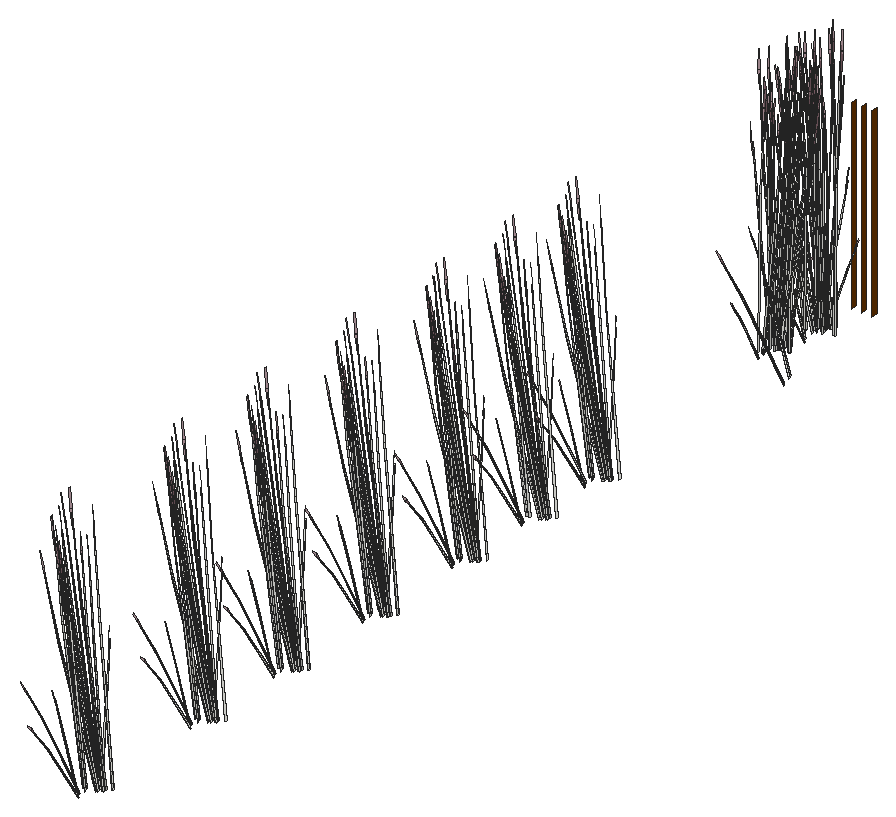
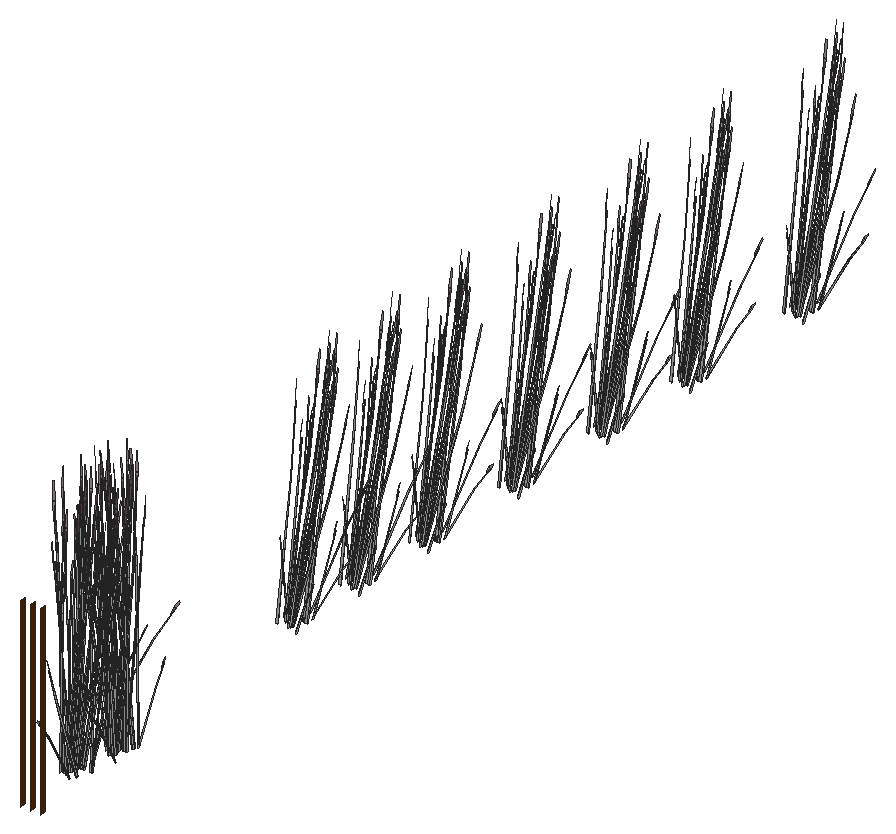
# SketchUp Ruby script. Lengths in inches.
U = 1.inch
M = Sketchup.active_model
def pt(a) = Geom::Point3d.new(a.map { |v| v * U })
def face(e, loops, mat)
  f = e.add_face(loops[0].map { |a| pt(a) })
  loops[1..].each { |l| e.add_face(l.map { |a| pt(a) }).erase! }
  f.material = f.back_material = mat if mat
  f
end
# faces: each face lists its corners as indices into pts; further lists are holes
def faces(e, pts, list, mat = nil) = list.each { |f| face(e, (f[0].is_a?(Array) ? f : [f]).map { |l| l.map { |i| pts[i] } }, mat) }
# xy, xz, yz: faces in a plane at the given z, y or x. An outline is a flat list of corners, or four numbers for a rectangle; further outlines are holes
def ring(l) = l.size == 4 ? [[l[0], l[1]], [l[2], l[1]], [l[2], l[3]], [l[0], l[3]]] : l.each_slice(2).to_a
def flat(e, list, mat, &to3) = list.each { |f| face(e, (f[0].is_a?(Array) ? f : [f]).map { |l| ring(l).map { |u, v| to3.(u, v) } }, mat) }
def xy(e, z, list, mat = nil) = flat(e, list, mat) { |x, y| [x, y, z] }
def xz(e, y, list, mat = nil) = flat(e, list, mat) { |x, z| [x, y, z] }
def yz(e, x, list, mat = nil) = flat(e, list, mat) { |y, z| [x, y, z] }
def lines(e, pts, list) = list.each { |a, b| e.add_line(pt(pts[a]), pt(pts[b])) }
# prism: a flat outline (further loops are holes) pulled along v
def prism(e, loops, v, mat = nil)
  f = face(e, loops, mat); d = Geom::Vector3d.new(v.map { |x| x * U })
  f.pushpull(f.normal.samedirection?(d) ? d.length : -d.length)
end
def box(e, o, s, mat = nil) = prism(e, [[o, [o[0] + s[0], o[1], o[2]], [o[0] + s[0], o[1] + s[1], o[2]], [o[0], o[1] + s[1], o[2]]]], [0, 0, s[2]], mat)
def at(x, y, z, deg = 0) = Geom::Transformation.translation(pt([x, y, z])) * Geom::Transformation.rotation(ORIGIN, Z_AXIS, deg.degrees)
def axes(o, x, y, z) = Geom::Transformation.new([*x, 0, *y, 0, *z, 0, *pt(o).to_a, 1])
def part(name) = M.definitions.add(name)
# library, detail: a bought-in or finely detailed component or shape, given as its bounding box
def library(name, o, s) = part(name).tap { |d| box(d.entities, o, s) }
def detail(e, o, s) = box(e.add_group.entities, o, s)
def put(e, d, t, mat = nil) = e.add_instance(d, t).tap { |i| i.material = mat if mat }
def group(e, t, mat = nil) = e.add_group.tap { |g| g.transformation = t; g.material = mat if mat }.entities
root = M.entities
M.materials.add("C08_Toffee_Ember").color = [102, 51, 0]
M.materials.add("LightPink_Translucent").color = [144, 107, 117]
M.materials["LightPink_Translucent"].alpha = 0.75
c1 = part("blade")
p = [[2.15,0.21,22],[0,0.17,0],[0.09,0.45,0],[2.18,0.31,22],[2.29,0.31,22],[0.38,0.45,0],
  [2.48,0.24,33],[2.49,0.24,33],[2.48,0.22,33]]
faces(c1.entities,p,[[0,1,2,3],[4,5,2,3],[6,3,4,7],[8,0,3,6]])
c2 = part("seeds")
p = [[0.3,-0.1,1.38],[-0.01,-0.03,1.59],[-0.01,-0.03,0.03],[0.14,-0.07,-0.07],[0.29,-0.03,3],[0.15,0.01,3.11]]
faces(c2.entities,p,[[0,1,2,3],[1,0,4,5]],"LightPink_Translucent")
c3 = part("blade with seeds")
put(c3.entities,c1,at(0,0,0))
put(c3.entities,c2,axes([2.4,0.25,30.99],[1.5799,-0.05474,1.17369],[-0.12525,1.92788,0.29478],[-0.07173,-0.02425,1.56792]))
yz(root,665.17,[[360,510,361,546]],"C08_Toffee_Ember")
yz(root,667.1875,[[360,510,361,546]],"C08_Toffee_Ember")
yz(root,669.21,[[360,510,361,546]],"C08_Toffee_Ember")
put(root,c3,axes([668.03,349.66,511.83],[-0.70648,0.03525,-0.37133],[-0.06389,-0.58508,0.17871],[-0.12647,0.0593,1.19224]))
put(root,c3,axes([666.41,341.29,512.17],[0.48065,0.34305,0.12018],[-0.40092,0.38703,-0.34318],[-0.1116,0.05232,1.05198]))
put(root,c3,axes([668.41,171,511.24],[0.08727,0.05704,1.46364],[0.14797,0.52853,-0.2236],[-0.19341,0.11271,0.24931]))
put(root,c3,axes([668.41,198.45,511.24],[0.08727,0.05704,1.46364],[0.14797,0.52853,-0.2236],[-0.19341,0.11271,0.24931]))
put(root,c3,axes([668.41,240.44,511.24],[0.08727,0.05704,1.46364],[0.14797,0.52853,-0.2236],[-0.19341,0.11271,0.24931]))
put(root,c3,axes([668.41,262.29,511.24],[0.08727,0.05704,1.46364],[0.14797,0.52853,-0.2236],[-0.19341,0.11271,0.24931]))
put(root,c3,axes([668.41,294.48,511.24],[0.08727,0.05704,1.46364],[0.14797,0.52853,-0.2236],[-0.19341,0.11271,0.24931]))
put(root,c3,axes([668.41,218.75,511.24],[0.08727,0.05704,1.46364],[0.14797,0.52853,-0.2236],[-0.19341,0.11271,0.24931]))
put(root,c3,axes([668.41,279.15,511.24],[0.08727,0.05704,1.46364],[0.14797,0.52853,-0.2236],[-0.19341,0.11271,0.24931]))
put(root,c3,axes([667.25,349.59,512.02],[0.17244,-0.67657,-0.19446],[0.81759,0.11793,0.42555],[-0.14286,-0.09343,1.29846]))
put(root,c3,axes([666.24,340.86,511.91],[-0.60515,-0.49144,-0.05089],[0.60552,-0.49174,0],[-0.02113,-0.01716,1.45724]))
put(root,c3,axes([667.55,349.75,512.17],[-0.12551,0.50956,0.12018],[-0.6132,-0.08845,-0.34318],[-0.1116,-0.05232,1.05198]))
put(root,c3,axes([666.57,342.38,511.93],[0.81449,0.18558,0.25528],[-0.20377,0.66335,-0.30288],[-0.13481,0.08302,1.36855]))
put(root,c3,axes([665.38,337.29,511.24],[-0.10912,0.02057,1.46364],[-0.60346,-0.23156,-0.2236],[0.01013,-0.19315,0.24931]))
put(root,c3,axes([668.77,351.17,511.67],[-0.60889,0.28548,-0.4121],[-0.36394,-0.51192,0],[-0.13868,0.06502,1.30728]))
put(root,c3,axes([665.16,348.32,511.67],[0,-0.57097,-0.4121],[0.72788,0,0],[0,-0.13004,1.30728]))
put(root,c3,axes([668.81,351.01,511.82],[-0.40169,-0.57414,-0.04268],[0.68052,-0.31907,0.42834],[-0.16769,0.05466,1.35813]))
put(root,c3,axes([665.02,340.3,511.96],[0.28286,0.63846,0.37976],[-0.80821,0.22202,0.14902],[0.00988,-0.11732,1.31851]))
put(root,c3,axes([664.89,340.22,511.83],[0.31565,-0.51449,-0.37133],[0.65588,0.24761,0.17871],[0,-0.1186,1.19224]))
put(root,c3,axes([665.7,341.875,511.83],[-0.21227,-0.49226,0],[0.60616,-0.17239,0],[0,0,1.28128]))
put(root,c3,axes([664.92,342.91,511.24],[0.10529,-0.03107,1.46364],[0.63335,0.17101,-0.2236],[0.01852,0.19274,0.24931]))
put(root,c3,axes([668.625,350.94,511.68],[-0.60696,-0.14127,-0.25712],[0.15283,-0.49751,0.25712],[-0.12236,0.05737,1.15348]))
put(root,c3,axes([667.07,348.98,512.21],[-0.73268,-0.27244,-0.24149],[0.35279,-0.57501,-0.41502],[-0.02303,-0.14118,1.32557]))
put(root,c3,axes([665.73,351.33,512.34],[0.59102,-0.10111,0.05401],[0.13587,0.40735,-0.71633],[-0.03747,0.2062,0.64209]))
put(root,c3,axes([668.52,349.5,512.21],[0.07581,0.65151,-0.24149],[-0.7896,0.03939,-0.41502],[-0.13904,0.08678,1.32557]))
put(root,c3,axes([666.55,340.9,511.83],[-0.31565,0.51449,-0.37133],[-0.65588,-0.24761,0.17871],[0,0.1186,1.19224]))
put(root,c3,axes([666.74,348.4,511.74],[-0.26718,-0.5855,-0.57963],[0.76964,-0.21087,-0.15213],[-0.02953,-0.19827,1.27944]))
put(root,c3,axes([670.77,169.29,511.71],[-0.67676,-0.09361,-0.51753],[0.14281,-0.57742,-0.13583],[-0.20196,-0.06997,1.14236]))
put(root,c3,axes([670.77,196.75,511.71],[-0.67676,-0.09361,-0.51753],[0.14281,-0.57742,-0.13583],[-0.20196,-0.06997,1.14236]))
put(root,c3,axes([670.77,238.74,511.71],[-0.67676,-0.09361,-0.51753],[0.14281,-0.57742,-0.13583],[-0.20196,-0.06997,1.14236]))
put(root,c3,axes([670.77,260.58,511.71],[-0.67676,-0.09361,-0.51753],[0.14281,-0.57742,-0.13583],[-0.20196,-0.06997,1.14236]))
put(root,c3,axes([670.77,292.78,511.71],[-0.67676,-0.09361,-0.51753],[0.14281,-0.57742,-0.13583],[-0.20196,-0.06997,1.14236]))
put(root,c3,axes([670.77,217.04,511.71],[-0.67676,-0.09361,-0.51753],[0.14281,-0.57742,-0.13583],[-0.20196,-0.06997,1.14236]))
put(root,c3,axes([670.77,277.44,511.71],[-0.67676,-0.09361,-0.51753],[0.14281,-0.57742,-0.13583],[-0.20196,-0.06997,1.14236]))
put(root,c3,axes([666.03,340.35,511.83],[0,-0.66065,0],[0.81352,0,0],[0,0,1.48949]))
put(root,c3,axes([665.48,348.34,511.68],[0.45414,-0.35624,-0.25712],[0.45414,0.35624,0.25712],[0,-0.11474,1.15348]))
put(root,c3,axes([665.28,340.47,512.02],[0.73304,0.27674,0.19974],[-0.35279,0.57501,0.41502],[0,-0.13255,1.3325]))
put(root,c3,axes([667.53,346.03,511.77],[-0.44958,0.32756,-0.03231],[-0.41194,-0.35875,-0.14649],[-0.029,-0.10165,0.48318]))
put(root,c3,axes([666.44,340.61,511.9],[0,0.66033,-0.04679],[-0.81352,0,0],[0,0.02075,1.48875]))
put(root,c3,axes([667.35,349.26,511.96],[0.82229,0.1203,0.37976],[-0.16734,0.67942,0.14902],[-0.12017,-0.06561,1.31851]))
put(root,c3,axes([666.05,341.89,511.9],[0.28286,0.65594,-0.0499],[-0.80821,0.22985,0],[0.00988,0.02291,1.42904]))
put(root,c3,axes([669.88,170.38,511.67],[-0.60889,-0.28548,-0.4121],[0.36394,-0.51192,0],[-0.13868,-0.06502,1.30728]))
put(root,c3,axes([669.88,197.84,511.67],[-0.60889,-0.28548,-0.4121],[0.36394,-0.51192,0],[-0.13868,-0.06502,1.30728]))
put(root,c3,axes([669.88,239.83,511.67],[-0.60889,-0.28548,-0.4121],[0.36394,-0.51192,0],[-0.13868,-0.06502,1.30728]))
put(root,c3,axes([669.88,261.68,511.67],[-0.60889,-0.28548,-0.4121],[0.36394,-0.51192,0],[-0.13868,-0.06502,1.30728]))
put(root,c3,axes([669.88,293.87,511.67],[-0.60889,-0.28548,-0.4121],[0.36394,-0.51192,0],[-0.13868,-0.06502,1.30728]))
put(root,c3,axes([669.88,218.13,511.67],[-0.60889,-0.28548,-0.4121],[0.36394,-0.51192,0],[-0.13868,-0.06502,1.30728]))
put(root,c3,axes([669.88,278.54,511.67],[-0.60889,-0.28548,-0.4121],[0.36394,-0.51192,0],[-0.13868,-0.06502,1.30728]))
put(root,c3,axes([669.61,166.13,511.24],[-0.06302,0.07522,1.46364],[-0.63686,0.16217,-0.2236],[-0.15385,-0.14752,0.24931]))
put(root,c3,axes([669.61,193.59,511.24],[-0.06302,0.07522,1.46364],[-0.63686,0.16217,-0.2236],[-0.15385,-0.14752,0.24931]))
put(root,c3,axes([669.61,235.58,511.24],[-0.06302,0.07522,1.46364],[-0.63686,0.16217,-0.2236],[-0.15385,-0.14752,0.24931]))
put(root,c3,axes([669.61,257.42,511.24],[-0.06302,0.07522,1.46364],[-0.63686,0.16217,-0.2236],[-0.15385,-0.14752,0.24931]))
put(root,c3,axes([669.61,289.62,511.24],[-0.06302,0.07522,1.46364],[-0.63686,0.16217,-0.2236],[-0.15385,-0.14752,0.24931]))
put(root,c3,axes([669.61,213.88,511.24],[-0.06302,0.07522,1.46364],[-0.63686,0.16217,-0.2236],[-0.15385,-0.14752,0.24931]))
put(root,c3,axes([669.61,274.28,511.24],[-0.06302,0.07522,1.46364],[-0.63686,0.16217,-0.2236],[-0.15385,-0.14752,0.24931]))
put(root,c3,axes([670.25,170.73,511.97],[-0.40676,0.57214,0],[-0.68052,-0.31907,-0.42834],[-0.15499,-0.07267,1.3588]))
put(root,c3,axes([670.25,198.1875,511.97],[-0.40676,0.57214,0],[-0.68052,-0.31907,-0.42834],[-0.15499,-0.07267,1.3588]))
put(root,c3,axes([670.25,240.18,511.97],[-0.40676,0.57214,0],[-0.68052,-0.31907,-0.42834],[-0.15499,-0.07267,1.3588]))
put(root,c3,axes([670.25,262.02,511.97],[-0.40676,0.57214,0],[-0.68052,-0.31907,-0.42834],[-0.15499,-0.07267,1.3588]))
put(root,c3,axes([670.25,294.21,511.97],[-0.40676,0.57214,0],[-0.68052,-0.31907,-0.42834],[-0.15499,-0.07267,1.3588]))
put(root,c3,axes([670.25,218.48,511.97],[-0.40676,0.57214,0],[-0.68052,-0.31907,-0.42834],[-0.15499,-0.07267,1.3588]))
put(root,c3,axes([670.25,278.88,511.97],[-0.40676,0.57214,0],[-0.68052,-0.31907,-0.42834],[-0.15499,-0.07267,1.3588]))
put(root,c3,axes([664.375,338.38,511.97],[-0.40676,-0.57214,0],[0.68052,-0.31907,-0.42834],[0.15499,-0.07267,1.3588]))
put(root,c3,axes([668.39,341.03,511.83],[-0.81312,-0.00457,-0.0413],[0,-0.63814,0.41452],[-0.02555,0.14527,1.31432]))
put(root,c3,axes([667.8,350.4375,511.82],[-0.65588,-0.25634,0],[0.31565,-0.53263,0],[0,0,1.35047]))
put(root,c3,axes([669.32,351.08,511.97],[0.40676,0.57214,0],[-0.68052,0.31907,-0.42834],[-0.15499,0.07267,1.3588]))
put(root,c3,axes([665.65,339.93,511.96],[-0.53943,0.51816,0.37976],[-0.64086,-0.4574,0.14902],[0.13005,-0.05171,1.31851]))
put(root,c3,axes([666.57,340.75,511.84],[0.45414,0.3688,0],[-0.45414,0.3688,0],[0,0,1.40491]))
put(root,c3,axes([666.29,342.11,511.83],[0.65588,0.25634,0],[-0.31565,0.53263,0],[0,0,1.45212]))
put(root,c3,axes([669.51,171.56,512.15],[0.2053,-0.09007,1.18691],[0.50689,0.27159,-0.25526],[-0.15087,0.235,0.50747]))
put(root,c3,axes([669.51,199.02,512.15],[0.2053,-0.09007,1.18691],[0.50689,0.27159,-0.25526],[-0.15087,0.235,0.50747]))
put(root,c3,axes([669.51,241,512.15],[0.2053,-0.09007,1.18691],[0.50689,0.27159,-0.25526],[-0.15087,0.235,0.50747]))
put(root,c3,axes([669.51,262.85,512.15],[0.2053,-0.09007,1.18691],[0.50689,0.27159,-0.25526],[-0.15087,0.235,0.50747]))
put(root,c3,axes([669.51,295.04,512.15],[0.2053,-0.09007,1.18691],[0.50689,0.27159,-0.25526],[-0.15087,0.235,0.50747]))
put(root,c3,axes([669.51,219.31,512.15],[0.2053,-0.09007,1.18691],[0.50689,0.27159,-0.25526],[-0.15087,0.235,0.50747]))
put(root,c3,axes([669.51,279.71,512.15],[0.2053,-0.09007,1.18691],[0.50689,0.27159,-0.25526],[-0.15087,0.235,0.50747]))
put(root,c3,axes([669.22,166.42,511.77],[-0.18768,0.46622,-0.03231],[-0.57763,-0.14342,-0.14649],[-0.0877,-0.07626,0.48318]))
put(root,c3,axes([669.22,193.88,511.77],[-0.18768,0.46622,-0.03231],[-0.57763,-0.14342,-0.14649],[-0.0877,-0.07626,0.48318]))
put(root,c3,axes([669.22,235.87,511.77],[-0.18768,0.46622,-0.03231],[-0.57763,-0.14342,-0.14649],[-0.0877,-0.07626,0.48318]))
put(root,c3,axes([669.22,257.71,511.77],[-0.18768,0.46622,-0.03231],[-0.57763,-0.14342,-0.14649],[-0.0877,-0.07626,0.48318]))
put(root,c3,axes([669.22,289.91,511.77],[-0.18768,0.46622,-0.03231],[-0.57763,-0.14342,-0.14649],[-0.0877,-0.07626,0.48318]))
put(root,c3,axes([669.22,214.17,511.77],[-0.18768,0.46622,-0.03231],[-0.57763,-0.14342,-0.14649],[-0.0877,-0.07626,0.48318]))
put(root,c3,axes([669.22,274.57,511.77],[-0.18768,0.46622,-0.03231],[-0.57763,-0.14342,-0.14649],[-0.0877,-0.07626,0.48318]))
put(root,c3,axes([668.67,349.625,512.17],[0.48065,0.34305,0.12018],[-0.40092,0.38703,-0.34318],[-0.1116,0.05232,1.05198]))
put(root,c3,axes([668.5,349.2,511.91],[-0.60515,-0.49144,-0.05089],[0.60552,-0.49174,0],[-0.02113,-0.01716,1.45724]))
put(root,c3,axes([666.35,340.2,511.98],[-0.82229,-0.1203,0.40835],[0.16734,-0.67942,0.16024],[0.12017,0.06561,1.41775]))
put(root,c3,axes([670.08,165.83,512.15],[-0.0394,0.18678,1.18691],[-0.57594,0.15636,-0.25526],[-0.13463,-0.24142,0.50747]))
put(root,c3,axes([670.08,193.29,512.15],[-0.0394,0.18678,1.18691],[-0.57594,0.15636,-0.25526],[-0.13463,-0.24142,0.50747]))
put(root,c3,axes([670.08,235.28,512.15],[-0.0394,0.18678,1.18691],[-0.57594,0.15636,-0.25526],[-0.13463,-0.24142,0.50747]))
put(root,c3,axes([670.08,257.125,512.15],[-0.0394,0.18678,1.18691],[-0.57594,0.15636,-0.25526],[-0.13463,-0.24142,0.50747]))
put(root,c3,axes([670.08,289.32,512.15],[-0.0394,0.18678,1.18691],[-0.57594,0.15636,-0.25526],[-0.13463,-0.24142,0.50747]))
put(root,c3,axes([670.08,213.58,512.15],[-0.0394,0.18678,1.18691],[-0.57594,0.15636,-0.25526],[-0.13463,-0.24142,0.50747]))
put(root,c3,axes([670.08,273.99,512.15],[-0.0394,0.18678,1.18691],[-0.57594,0.15636,-0.25526],[-0.13463,-0.24142,0.50747]))
put(root,c3,axes([668.22,341.125,511.68],[-0.45414,0.35624,-0.25712],[-0.45414,-0.35624,0.25712],[0,0.11474,1.15348]))
put(root,c3,axes([668.83,350.72,511.93],[0.81449,0.18558,0.25528],[-0.20377,0.66335,-0.30288],[-0.13481,0.08302,1.36855]))
put(root,c3,axes([667.64,345.63,511.24],[-0.10912,0.02057,1.46364],[-0.60346,-0.23156,-0.2236],[0.01013,-0.19315,0.24931]))
put(root,c3,axes([671.53,169.38,512.21],[-0.65687,0.37907,-0.24149],[-0.43681,-0.53562,-0.41502],[-0.16207,-0.0544,1.32557]))
put(root,c3,axes([671.53,196.83,512.21],[-0.65687,0.37907,-0.24149],[-0.43681,-0.53562,-0.41502],[-0.16207,-0.0544,1.32557]))
put(root,c3,axes([671.53,238.82,512.21],[-0.65687,0.37907,-0.24149],[-0.43681,-0.53562,-0.41502],[-0.16207,-0.0544,1.32557]))
put(root,c3,axes([671.53,260.67,512.21],[-0.65687,0.37907,-0.24149],[-0.43681,-0.53562,-0.41502],[-0.16207,-0.0544,1.32557]))
put(root,c3,axes([671.53,292.86,512.21],[-0.65687,0.37907,-0.24149],[-0.43681,-0.53562,-0.41502],[-0.16207,-0.0544,1.32557]))
put(root,c3,axes([671.53,217.125,512.21],[-0.65687,0.37907,-0.24149],[-0.43681,-0.53562,-0.41502],[-0.16207,-0.0544,1.32557]))
put(root,c3,axes([671.53,277.53,512.21],[-0.65687,0.37907,-0.24149],[-0.43681,-0.53562,-0.41502],[-0.16207,-0.0544,1.32557]))
put(root,c3,axes([666.92,341.06,511.74],[0.23855,0.52277,-0.57446],[-0.68718,0.18827,-0.15077],[0.02637,0.17702,1.26801]))
put(root,c3,axes([666.59,340.5,511.83],[0.72788,0,0],[0,0.59111,0],[0,0,1.48078]))
put(root,c3,axes([667.27,348.64,511.96],[0.28286,0.63846,0.37976],[-0.80821,0.22202,0.14902],[0.00988,-0.11732,1.31851]))
put(root,c3,axes([668.91,168.55,511.97],[-0.81352,0,0],[0,-0.63814,-0.42834],[0,-0.14534,1.3588]))
put(root,c3,axes([668.91,196.01,511.97],[-0.81352,0,0],[0,-0.63814,-0.42834],[0,-0.14534,1.3588]))
put(root,c3,axes([668.91,216.3,511.97],[-0.81352,0,0],[0,-0.63814,-0.42834],[0,-0.14534,1.3588]))
put(root,c3,axes([668.91,238,511.97],[-0.81352,0,0],[0,-0.63814,-0.42834],[0,-0.14534,1.3588]))
put(root,c3,axes([668.91,259.84,511.97],[-0.81352,0,0],[0,-0.63814,-0.42834],[0,-0.14534,1.3588]))
put(root,c3,axes([668.91,276.7,511.97],[-0.81352,0,0],[0,-0.63814,-0.42834],[0,-0.14534,1.3588]))
put(root,c3,axes([668.91,292.04,511.97],[-0.81352,0,0],[0,-0.63814,-0.42834],[0,-0.14534,1.3588]))
put(root,c3,axes([667.14,348.56,511.83],[0.31565,-0.51449,-0.37133],[0.65588,0.24761,0.17871],[0,-0.1186,1.19224]))
put(root,c3,axes([670.05,170.17,511.68],[-0.15283,-0.49751,-0.25712],[0.60696,-0.14127,0.25712],[-0.12236,-0.05737,1.15348]))
put(root,c3,axes([670.05,197.63,511.68],[-0.15283,-0.49751,-0.25712],[0.60696,-0.14127,0.25712],[-0.12236,-0.05737,1.15348]))
put(root,c3,axes([670.05,239.62,511.68],[-0.15283,-0.49751,-0.25712],[0.60696,-0.14127,0.25712],[-0.12236,-0.05737,1.15348]))
put(root,c3,axes([670.05,261.46,511.68],[-0.15283,-0.49751,-0.25712],[0.60696,-0.14127,0.25712],[-0.12236,-0.05737,1.15348]))
put(root,c3,axes([670.05,293.66,511.68],[-0.15283,-0.49751,-0.25712],[0.60696,-0.14127,0.25712],[-0.12236,-0.05737,1.15348]))
put(root,c3,axes([670.05,217.92,511.68],[-0.15283,-0.49751,-0.25712],[0.60696,-0.14127,0.25712],[-0.12236,-0.05737,1.15348]))
put(root,c3,axes([670.05,278.32,511.68],[-0.15283,-0.49751,-0.25712],[0.60696,-0.14127,0.25712],[-0.12236,-0.05737,1.15348]))
put(root,c3,axes([665.18,339.96,512.21],[-0.07581,-0.65151,-0.24149],[0.7896,-0.03939,-0.41502],[0.13904,-0.08678,1.32557]))
put(root,c3,axes([666.84,340.4375,512.17],[0.60616,-0.16651,0.12018],[0.21227,0.47548,-0.34318],[0,0.10465,1.05198]))
put(root,c3,axes([667.95,350.22,511.83],[-0.21227,-0.49226,0],[0.60616,-0.17239,0],[0,0,1.28128]))
put(root,c3,axes([667.18,351.25,511.24],[0.10529,-0.03107,1.46364],[0.63335,0.17101,-0.2236],[0.01852,0.19274,0.24931]))
put(root,c3,axes([666.63,340.48,512.21],[0.73268,0.27244,-0.24149],[-0.35279,0.57501,-0.41502],[0.02303,0.14118,1.32557]))
put(root,c3,axes([671.97,169.79,511.71],[-0.43821,0.42916,-0.51753],[-0.54436,-0.38915,-0.13583],[-0.1756,0.10706,1.14236]))
put(root,c3,axes([671.97,197.25,511.71],[-0.43821,0.42916,-0.51753],[-0.54436,-0.38915,-0.13583],[-0.1756,0.10706,1.14236]))
put(root,c3,axes([671.97,217.54,511.71],[-0.43821,0.42916,-0.51753],[-0.54436,-0.38915,-0.13583],[-0.1756,0.10706,1.14236]))
put(root,c3,axes([671.97,239.24,511.71],[-0.43821,0.42916,-0.51753],[-0.54436,-0.38915,-0.13583],[-0.1756,0.10706,1.14236]))
put(root,c3,axes([671.97,261.08,511.71],[-0.43821,0.42916,-0.51753],[-0.54436,-0.38915,-0.13583],[-0.1756,0.10706,1.14236]))
put(root,c3,axes([671.97,277.94,511.71],[-0.43821,0.42916,-0.51753],[-0.54436,-0.38915,-0.13583],[-0.1756,0.10706,1.14236]))
put(root,c3,axes([671.97,293.28,511.71],[-0.43821,0.42916,-0.51753],[-0.54436,-0.38915,-0.13583],[-0.1756,0.10706,1.14236]))
put(root,c3,axes([665.07,338.52,511.68],[0.60696,0.14127,-0.25712],[-0.15283,0.49751,0.25712],[0.12236,-0.05737,1.15348]))
put(root,c3,axes([669.54,168.38,511.93],[-0.60515,0.48003,0.25528],[-0.60552,-0.47498,-0.30288],[-0.02113,-0.13632,1.36855]))
put(root,c3,axes([669.54,195.84,511.93],[-0.60515,0.48003,0.25528],[-0.60552,-0.47498,-0.30288],[-0.02113,-0.13632,1.36855]))
put(root,c3,axes([669.54,216.13,511.93],[-0.60515,0.48003,0.25528],[-0.60552,-0.47498,-0.30288],[-0.02113,-0.13632,1.36855]))
put(root,c3,axes([669.54,237.83,511.93],[-0.60515,0.48003,0.25528],[-0.60552,-0.47498,-0.30288],[-0.02113,-0.13632,1.36855]))
put(root,c3,axes([669.54,259.67,511.93],[-0.60515,0.48003,0.25528],[-0.60552,-0.47498,-0.30288],[-0.02113,-0.13632,1.36855]))
put(root,c3,axes([669.54,276.53,511.93],[-0.60515,0.48003,0.25528],[-0.60552,-0.47498,-0.30288],[-0.02113,-0.13632,1.36855]))
put(root,c3,axes([669.54,291.87,511.93],[-0.60515,0.48003,0.25528],[-0.60552,-0.47498,-0.30288],[-0.02113,-0.13632,1.36855]))
put(root,c3,axes([668.81,349.24,511.83],[-0.31565,0.51449,-0.37133],[-0.65588,-0.24761,0.17871],[0,0.1186,1.19224]))
put(root,c3,axes([672.27,169.55,512.05],[-0.63528,-0.45956,-0.20909],[0.53456,-0.51604,0.45758],[-0.17107,0.05376,1.39619]))
put(root,c3,axes([672.27,197.01,512.05],[-0.63528,-0.45956,-0.20909],[0.53456,-0.51604,0.45758],[-0.17107,0.05376,1.39619]))
put(root,c3,axes([672.27,239,512.05],[-0.63528,-0.45956,-0.20909],[0.53456,-0.51604,0.45758],[-0.17107,0.05376,1.39619]))
put(root,c3,axes([672.27,260.84,512.05],[-0.63528,-0.45956,-0.20909],[0.53456,-0.51604,0.45758],[-0.17107,0.05376,1.39619]))
put(root,c3,axes([672.27,293.04,512.05],[-0.63528,-0.45956,-0.20909],[0.53456,-0.51604,0.45758],[-0.17107,0.05376,1.39619]))
put(root,c3,axes([672.27,217.3,512.05],[-0.63528,-0.45956,-0.20909],[0.53456,-0.51604,0.45758],[-0.17107,0.05376,1.39619]))
put(root,c3,axes([672.27,277.7,512.05],[-0.63528,-0.45956,-0.20909],[0.53456,-0.51604,0.45758],[-0.17107,0.05376,1.39619]))
put(root,c3,axes([668.53,341.14,511.67],[0,0.57097,-0.4121],[-0.72788,0,0],[0,0.13004,1.30728]))
put(root,c3,axes([671.12,169.11,511.83],[-0.39083,-0.47924,-0.37133],[0.59199,-0.33747,0.17871],[-0.12647,-0.0593,1.19224]))
put(root,c3,axes([671.12,196.57,511.83],[-0.39083,-0.47924,-0.37133],[0.59199,-0.33747,0.17871],[-0.12647,-0.0593,1.19224]))
put(root,c3,axes([671.12,238.55,511.83],[-0.39083,-0.47924,-0.37133],[0.59199,-0.33747,0.17871],[-0.12647,-0.0593,1.19224]))
put(root,c3,axes([671.12,260.4,511.83],[-0.39083,-0.47924,-0.37133],[0.59199,-0.33747,0.17871],[-0.12647,-0.0593,1.19224]))
put(root,c3,axes([671.12,292.59,511.83],[-0.39083,-0.47924,-0.37133],[0.59199,-0.33747,0.17871],[-0.12647,-0.0593,1.19224]))
put(root,c3,axes([671.12,216.86,511.83],[-0.39083,-0.47924,-0.37133],[0.59199,-0.33747,0.17871],[-0.12647,-0.0593,1.19224]))
put(root,c3,axes([671.12,277.26,511.83],[-0.39083,-0.47924,-0.37133],[0.59199,-0.33747,0.17871],[-0.12647,-0.0593,1.19224]))
put(root,c3,axes([664.93,338.29,511.67],[0.60889,-0.28548,-0.4121],[0.36394,0.51192,0],[0.13868,-0.06502,1.30728]))
put(root,c3,axes([673.62,334.13,512.15],[0.2261,0.04687,1.18691],[0.14573,0.47875,-0.25526],[-0.30712,0.08962,0.50747]))
put(root,c3,axes([668.29,348.69,511.83],[0,-0.66065,0],[0.81352,0,0],[0,0,1.48949]))
put(root,c3,axes([666.15,339.71,512.17],[0.12551,-0.50956,0.12018],[0.6132,0.08845,-0.34318],[0.1116,0.05232,1.05198]))
put(root,c3,axes([667.54,348.8125,512.02],[0.73304,0.27674,0.19974],[-0.35279,0.57501,0.41502],[0,-0.13255,1.3325]))
put(root,c3,axes([668.7,348.95,511.9],[0,0.66033,-0.04679],[-0.81352,0,0],[0,0.02075,1.48875]))
put(root,c3,axes([671.95,169.45,511.83],[-0.70648,0.03525,-0.37133],[-0.06389,-0.58508,0.17871],[-0.12647,0.0593,1.19224]))
put(root,c3,axes([671.95,196.91,511.83],[-0.70648,0.03525,-0.37133],[-0.06389,-0.58508,0.17871],[-0.12647,0.0593,1.19224]))
put(root,c3,axes([671.95,238.9,511.83],[-0.70648,0.03525,-0.37133],[-0.06389,-0.58508,0.17871],[-0.12647,0.0593,1.19224]))
put(root,c3,axes([671.95,260.74,511.83],[-0.70648,0.03525,-0.37133],[-0.06389,-0.58508,0.17871],[-0.12647,0.0593,1.19224]))
put(root,c3,axes([671.95,292.9375,511.83],[-0.70648,0.03525,-0.37133],[-0.06389,-0.58508,0.17871],[-0.12647,0.0593,1.19224]))
put(root,c3,axes([671.95,217.2,511.83],[-0.70648,0.03525,-0.37133],[-0.06389,-0.58508,0.17871],[-0.12647,0.0593,1.19224]))
put(root,c3,axes([671.95,277.6,511.83],[-0.70648,0.03525,-0.37133],[-0.06389,-0.58508,0.17871],[-0.12647,0.0593,1.19224]))
put(root,c3,axes([668.3125,350.23,511.9],[0.28286,0.65594,-0.0499],[-0.80821,0.22985,0],[0.00988,0.02291,1.42904]))
put(root,c3,axes([666.49,341.81,511.8125],[0.68303,-0.19373,-0.15934],[0.24001,0.55805,0.00007],[0.07539,-0.02141,1.44335]))
put(root,c3,axes([666.63,346.72,511.97],[-0.40676,-0.57214,0],[0.68052,-0.31907,-0.42834],[0.15499,-0.07267,1.3588]))
put(root,c3,axes([671.17,169.38,512.02],[0.17244,-0.67657,-0.19446],[0.81759,0.11793,0.42555],[-0.14286,-0.09343,1.29846]))
put(root,c3,axes([671.17,196.84,512.02],[0.17244,-0.67657,-0.19446],[0.81759,0.11793,0.42555],[-0.14286,-0.09343,1.29846]))
put(root,c3,axes([671.17,217.13,512.02],[0.17244,-0.67657,-0.19446],[0.81759,0.11793,0.42555],[-0.14286,-0.09343,1.29846]))
put(root,c3,axes([671.17,238.83,512.02],[0.17244,-0.67657,-0.19446],[0.81759,0.11793,0.42555],[-0.14286,-0.09343,1.29846]))
put(root,c3,axes([671.17,260.67,512.02],[0.17244,-0.67657,-0.19446],[0.81759,0.11793,0.42555],[-0.14286,-0.09343,1.29846]))
put(root,c3,axes([671.17,277.53,512.02],[0.17244,-0.67657,-0.19446],[0.81759,0.11793,0.42555],[-0.14286,-0.09343,1.29846]))
put(root,c3,axes([671.17,292.87,512.02],[0.17244,-0.67657,-0.19446],[0.81759,0.11793,0.42555],[-0.14286,-0.09343,1.29846]))
put(root,c3,axes([670.65,349.37,511.83],[-0.81312,-0.00457,-0.0413],[0,-0.63814,0.41452],[-0.02555,0.14527,1.31432]))
put(root,c3,axes([671.47,169.54,512.17],[-0.12551,0.50956,0.12018],[-0.6132,-0.08845,-0.34318],[-0.1116,-0.05232,1.05198]))
put(root,c3,axes([671.47,197,512.17],[-0.12551,0.50956,0.12018],[-0.6132,-0.08845,-0.34318],[-0.1116,-0.05232,1.05198]))
put(root,c3,axes([671.47,238.99,512.17],[-0.12551,0.50956,0.12018],[-0.6132,-0.08845,-0.34318],[-0.1116,-0.05232,1.05198]))
put(root,c3,axes([671.47,260.83,512.17],[-0.12551,0.50956,0.12018],[-0.6132,-0.08845,-0.34318],[-0.1116,-0.05232,1.05198]))
put(root,c3,axes([671.47,293.03,512.17],[-0.12551,0.50956,0.12018],[-0.6132,-0.08845,-0.34318],[-0.1116,-0.05232,1.05198]))
put(root,c3,axes([671.47,217.29,512.17],[-0.12551,0.50956,0.12018],[-0.6132,-0.08845,-0.34318],[-0.1116,-0.05232,1.05198]))
put(root,c3,axes([671.47,277.69,512.17],[-0.12551,0.50956,0.12018],[-0.6132,-0.08845,-0.34318],[-0.1116,-0.05232,1.05198]))
put(root,c3,axes([674.49,331.8125,512.15],[0.12702,0.15896,1.18691],[-0.2927,0.4321,-0.25526],[-0.30054,-0.10328,0.50747]))
put(root,c3,axes([672.69,170.96,511.67],[-0.60889,0.28548,-0.4121],[-0.36394,-0.51192,0],[-0.13868,0.06502,1.30728]))
put(root,c3,axes([672.69,198.42,511.67],[-0.60889,0.28548,-0.4121],[-0.36394,-0.51192,0],[-0.13868,0.06502,1.30728]))
put(root,c3,axes([672.69,240.41,511.67],[-0.60889,0.28548,-0.4121],[-0.36394,-0.51192,0],[-0.13868,0.06502,1.30728]))
put(root,c3,axes([672.69,262.25,511.67],[-0.60889,0.28548,-0.4121],[-0.36394,-0.51192,0],[-0.13868,0.06502,1.30728]))
put(root,c3,axes([672.69,294.45,511.67],[-0.60889,0.28548,-0.4121],[-0.36394,-0.51192,0],[-0.13868,0.06502,1.30728]))
put(root,c3,axes([672.69,218.71,511.67],[-0.60889,0.28548,-0.4121],[-0.36394,-0.51192,0],[-0.13868,0.06502,1.30728]))
put(root,c3,axes([672.69,279.11,511.67],[-0.60889,0.28548,-0.4121],[-0.36394,-0.51192,0],[-0.13868,0.06502,1.30728]))
put(root,c3,axes([666.5,340.15,511.83],[0.39083,0.47924,-0.37133],[-0.59199,0.33747,0.17871],[0.12647,0.0593,1.19224]))
put(root,c3,axes([669.09,168.12,511.67],[0,-0.57097,-0.4121],[0.72788,0,0],[0,-0.13004,1.30728]))
put(root,c3,axes([669.09,195.57,511.67],[0,-0.57097,-0.4121],[0.72788,0,0],[0,-0.13004,1.30728]))
put(root,c3,axes([669.09,237.5625,511.67],[0,-0.57097,-0.4121],[0.72788,0,0],[0,-0.13004,1.30728]))
put(root,c3,axes([669.09,259.41,511.67],[0,-0.57097,-0.4121],[0.72788,0,0],[0,-0.13004,1.30728]))
put(root,c3,axes([669.09,291.6,511.67],[0,-0.57097,-0.4121],[0.72788,0,0],[0,-0.13004,1.30728]))
put(root,c3,axes([669.09,215.87,511.67],[0,-0.57097,-0.4121],[0.72788,0,0],[0,-0.13004,1.30728]))
